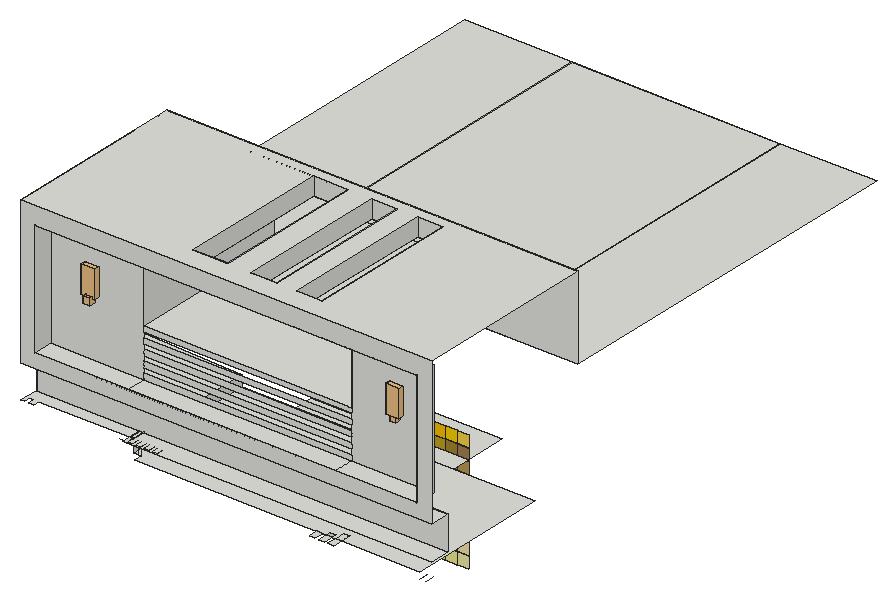
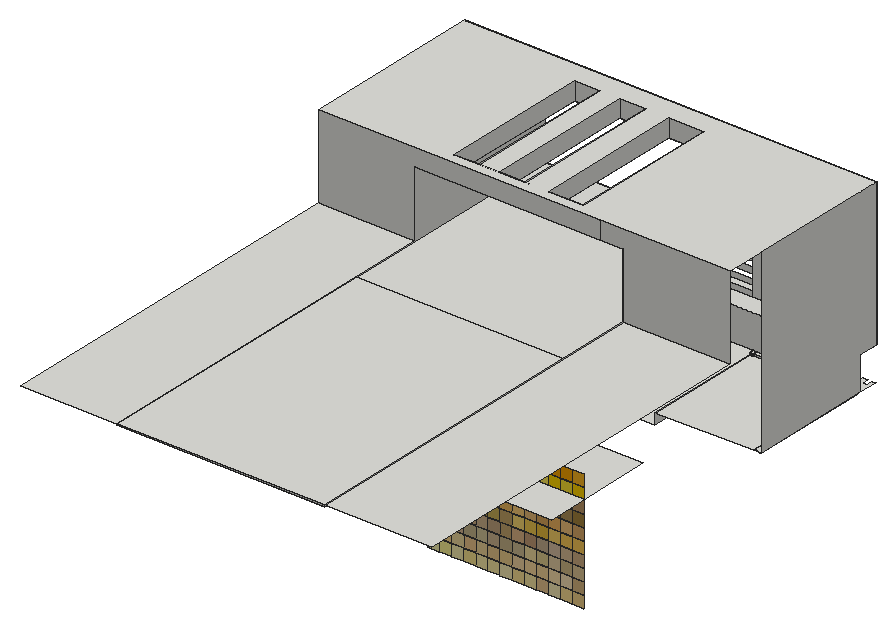
# SketchUp Ruby script. Lengths in inches.
U = 1.inch
M = Sketchup.active_model
def pt(a) = Geom::Point3d.new(a.map { |v| v * U })
def face(e, loops, mat)
  f = e.add_face(loops[0].map { |a| pt(a) })
  loops[1..].each { |l| e.add_face(l.map { |a| pt(a) }).erase! }
  f.material = f.back_material = mat if mat
  f
end
# faces: each face lists its corners as indices into pts; further lists are holes
def faces(e, pts, list, mat = nil) = list.each { |f| face(e, (f[0].is_a?(Array) ? f : [f]).map { |l| l.map { |i| pts[i] } }, mat) }
# xy, xz, yz: faces in a plane at the given z, y or x. An outline is a flat list of corners, or four numbers for a rectangle; further outlines are holes
def ring(l) = l.size == 4 ? [[l[0], l[1]], [l[2], l[1]], [l[2], l[3]], [l[0], l[3]]] : l.each_slice(2).to_a
def flat(e, list, mat, &to3) = list.each { |f| face(e, (f[0].is_a?(Array) ? f : [f]).map { |l| ring(l).map { |u, v| to3.(u, v) } }, mat) }
def xy(e, z, list, mat = nil) = flat(e, list, mat) { |x, y| [x, y, z] }
def xz(e, y, list, mat = nil) = flat(e, list, mat) { |x, z| [x, y, z] }
def yz(e, x, list, mat = nil) = flat(e, list, mat) { |y, z| [x, y, z] }
def lines(e, pts, list) = list.each { |a, b| e.add_line(pt(pts[a]), pt(pts[b])) }
# prism: a flat outline (further loops are holes) pulled along v
def prism(e, loops, v, mat = nil)
  f = face(e, loops, mat); d = Geom::Vector3d.new(v.map { |x| x * U })
  f.pushpull(f.normal.samedirection?(d) ? d.length : -d.length)
end
def box(e, o, s, mat = nil) = prism(e, [[o, [o[0] + s[0], o[1], o[2]], [o[0] + s[0], o[1] + s[1], o[2]], [o[0], o[1] + s[1], o[2]]]], [0, 0, s[2]], mat)
def at(x, y, z, deg = 0) = Geom::Transformation.translation(pt([x, y, z])) * Geom::Transformation.rotation(ORIGIN, Z_AXIS, deg.degrees)
def axes(o, x, y, z) = Geom::Transformation.new([*x, 0, *y, 0, *z, 0, *pt(o).to_a, 1])
def part(name) = M.definitions.add(name)
# library, detail: a bought-in or finely detailed component or shape, given as its bounding box
def library(name, o, s) = part(name).tap { |d| box(d.entities, o, s) }
def detail(e, o, s) = box(e.add_group.entities, o, s)
def put(e, d, t, mat = nil) = e.add_instance(d, t).tap { |i| i.material = mat if mat }
def group(e, t, mat = nil) = e.add_group.tap { |g| g.transformation = t; g.material = mat if mat }.entities
root = M.entities
M.materials.add("SW 0012 Empire Gold").color = [192, 162, 108]
M.materials.add("SW 0030 Colonial Yellow").color = [235, 202, 133]
M.materials.add("SW 0043 Peristyle Brass").color = [171, 151, 98]
M.materials.add("SW 0044 Hubbard Squash").color = [228, 196, 137]
M.materials.add("SW 0067 Belvedere Cream").color = [236, 208, 158]
M.materials.add("SW 0078 Sunbeam Yellow").color = [236, 216, 155]
M.materials.add("SW 2813 Downing Straw").color = [196, 173, 119]
M.materials.add("SW 2814 Rookwood Antique Gold").color = [158, 131, 78]
M.materials.add("SW 2817 Rookwood Amber").color = [185, 135, 62]
M.materials.add("SW 2831 Classical Gold").color = [230, 191, 112]
M.materials.add("SW 2834 Birdseye Maple").color = [221, 199, 142]
M.materials.add("SW 2853 New Colonial Yellow").color = [211, 178, 125]
M.materials.add("SW 2857 Peace Yellow").color = [231, 210, 153]
M.materials.add("SW 2858 Harvest Gold").color = [215, 167, 103]
M.materials.add("SW 2865 Classical Yellow").color = [244, 218, 144]
M.materials.add("SW 6114 Bagel").color = [213, 185, 146]
M.materials.add("SW 6115 Totally Tan").color = [202, 170, 129]
M.materials.add("SW 6116 Tatami Tan").color = [184, 148, 100]
M.materials.add("SW 6117 Smokey Topaz").color = [164, 127, 83]
M.materials.add("SW 6118 Leather Bound").color = [139, 102, 57]
M.materials.add("SW 6121 Whole Wheat").color = [203, 185, 145]
M.materials.add("SW 6122 Camelback").color = [194, 175, 133]
M.materials.add("SW 6123 Baguette").color = [175, 151, 103]
M.materials.add("SW 6128 Blonde").color = [217, 193, 145]
M.materials.add("SW 6129 Restrained Gold").color = [206, 183, 131]
M.materials.add("SW 6130 Mannered Gold").color = [189, 159, 99]
M.materials.add("SW 6131 Chamois").color = [172, 141, 84]
M.materials.add("SW 6132 Relic Bronze").color = [143, 113, 59]
M.materials.add("SW 6135 Ecru").color = [206, 193, 149]
M.materials.add("SW 6136 Harmonic Tan").color = [194, 179, 136]
M.materials.add("SW 6137 Burlap").color = [170, 155, 114]
M.materials.add("SW 6138 Artifact").color = [151, 136, 95]
M.materials.add("SW 6139 Mossy Gold").color = [124, 107, 64]
M.materials.add("SW 6366 Ambitious Amber").color = [238, 208, 148]
M.materials.add("SW 6367 Viva Gold").color = [227, 182, 114]
M.materials.add("SW 6368 Bakelite Gold").color = [212, 162, 89]
M.materials.add("SW 6369 Tassel").color = [195, 143, 67]
M.materials.add("SW 6370 Saucy Gold").color = [179, 122, 51]
M.materials.add("SW 6373 Harvester").color = [232, 201, 137]
M.materials.add("SW 6374 Torchlight").color = [226, 185, 106]
M.materials.add("SW 6375 Honeycomb").color = [210, 161, 84]
M.materials.add("SW 6376 Gold Coast").color = [195, 143, 57]
M.materials.add("SW 6377 Butterscotch").color = [180, 128, 52]
M.materials.add("SW 6380 Humble Gold").color = [232, 206, 147]
M.materials.add("SW 6381 Anjou Pear").color = [217, 181, 105]
M.materials.add("SW 6382 Ceremonial Gold").color = [208, 167, 85]
M.materials.add("SW 6383 Golden Rule").color = [199, 153, 65]
M.materials.add("SW 6384 Cut The Mustard").color = [182, 135, 47]
M.materials.add("SW 6388 Golden Fleece").color = [227, 182, 114]
M.materials.add("SW 6389 Butternut").color = [200, 164, 90]
M.materials.add("SW 6390 Bosc Pear").color = [188, 151, 83]
M.materials.add("SW 6391 Gallant Gold").color = [161, 128, 61]
M.materials.add("SW 6394 Sequin").color = [220, 200, 139]
M.materials.add("SW 6395 Alchemy").color = [197, 171, 86]
M.materials.add("SW 6396 Different Gold").color = [183, 156, 75]
M.materials.add("SW 6397 Nankeen").color = [162, 135, 46]
M.materials.add("SW 6398 Sconce Gold").color = [151, 121, 51]
M.materials.add("SW 6659 Captivating Cream").color = [243, 220, 176]
M.materials.add("SW 6660 Honey Blush").color = [243, 211, 152]
M.materials.add("SW 6661 Papaya").color = [238, 189, 120]
M.materials.add("SW 6662 Summer Day").color = [234, 176, 94]
M.materials.add("SW 6663 Saffron Thread").color = [223, 158, 74]
M.materials.add("SW 6666 Enjoyable Yellow").color = [244, 218, 167]
M.materials.add("SW 6667 Afterglow").color = [243, 209, 138]
M.materials.add("SW 6668 Sunrise").color = [242, 197, 116]
M.materials.add("SW 6669 Yarrow").color = [231, 180, 89]
M.materials.add("SW 6670 Gold Crest").color = [221, 159, 46]
M.materials.add("SW 6671 Curry").color = [214, 148, 38]
M.materials.add("SW 6673 Banana Cream").color = [243, 226, 174]
M.materials.add("SW 6674 Jonquil").color = [244, 216, 142]
M.materials.add("SW 6675 Afternoon").color = [248, 209, 116]
M.materials.add("SW 6676 Butterfield").color = [244, 196, 86]
M.materials.add("SW 6677 Goldenrod").color = [244, 196, 86]
M.materials.add("SW 6678 Sunflower").color = [223, 162, 35]
M.materials.add("SW 6680 Friendly Yellow").color = [241, 228, 176]
M.materials.add("SW 6681 Butter Up").color = [243, 225, 159]
M.materials.add("SW 6682 June Day").color = [242, 210, 111]
M.materials.add("SW 6683 Bee").color = [235, 196, 79]
M.materials.add("SW 6684 Brittlebush").color = [228, 184, 61]
M.materials.add("SW 6685 Trinket").color = [209, 161, 37]
M.materials.add("SW 6687 Lantern Light").color = [241, 228, 173]
M.materials.add("SW 6688 Solaria").color = [242, 221, 140]
M.materials.add("SW 6689 Overjoy").color = [233, 203, 89]
M.materials.add("SW 6690 Gambol Gold").color = [220, 186, 63]
M.materials.add("SW 6691 Glitzy Gold").color = [208, 168, 18]
M.materials.add("SW 6692 Auric").color = [191, 145, 0]
M.materials.add("SW 6694 Glad Yellow").color = [240, 230, 169]
M.materials.add("SW 6695 Midday").color = [242, 222, 135]
M.materials.add("SW 6696 Quilt Gold").color = [227, 203, 95]
M.materials.add("SW 6697 Nugget").color = [211, 184, 67]
M.materials.add("SW 6698 Kingdom Gold").color = [202, 173, 37]
M.materials.add("SW 6699 Crispy Gold").color = [191, 161, 37]
M.materials.add("SW 6888 Pizazz Peach").color = [243, 202, 146]
M.materials.add("SW 6889 Stirring Orange").color = [243, 181, 96]
M.materials.add("SW 6890 Osage Orange").color = [243, 166, 60]
M.materials.add("SW 6894 Forceful Orange").color = [242, 160, 0]
M.materials.add("SW 6895 Laughing Orange").color = [242, 160, 0]
M.materials.add("SW 6896 Solé").color = [243, 226, 157]
M.materials.add("SW 6897 Sundance").color = [245, 206, 103]
M.materials.add("SW 6898 Social Butterfly").color = [247, 193, 71]
M.materials.add("SW 6899 Nasturtiumb").color = [246, 178, 33]
M.materials.add("SW 6900 Optimistic Yellow").color = [242, 228, 163]
M.materials.add("SW 6901 Daffodil").color = [246, 223, 119]
M.materials.add("SW 6902 Decisive Yellow").color = [248, 211, 68]
M.materials.add("SW 6903 Cheerful").color = [250, 208, 0]
M.materials.add("SW 6904 Gusto Gold").color = [245, 181, 0]
M.materials.add("SW 6905 Goldfinch").color = [249, 192, 0]
M.materials.add("SW 6906 Citrus").color = [251, 205, 0]
M.materials.add("SW 6907 Forsythia").color = [251, 210, 0]
M.materials.add("SW 6908 Fun Yellow").color = [242, 235, 145]
M.materials.add("SW 6909 Lemon Twist").color = [248, 227, 86]
M.materials.add("SW 6910 Daisy").color = [246, 220, 49]
M.materials.add("SW 6911 Confident Yellow").color = [245, 214, 0]
M.materials.add("SW 6912 Glisten Yellow").color = [240, 235, 169]
M.materials.add("SW 7677 Gold Vessel").color = [233, 187, 138]
M.materials.add("SW 7679 Golden Gate").color = [217, 176, 132]
M.materials.add("SW 7680 Lanyard").color = [191, 153, 116]
M.materials.add("SW 7682 Bee_s Wax").color = [233, 192, 136]
M.materials.add("SW 7685 White Raisin").color = [228, 192, 140]
M.materials.add("SW 7689 Row House Tan").color = [211, 187, 159]
M.materials.add("SW 7690 Townhall Tan").color = [194, 171, 140]
M.materials.add("SW 7691 Biltmore Buff").color = [225, 202, 161]
M.materials.add("SW 7692 Cupola Yellow").color = [219, 188, 144]
M.materials.add("SW 7693 Stonebriar").color = [203, 172, 128]
M.materials.add("SW 7694 Dromedary Camel").color = [203, 175, 136]
M.materials.add("SW 7695 Mesa Tan").color = [190, 160, 124]
M.materials.add("SW 7697 Safari").color = [203, 179, 141]
M.materials.add("SW 7699 Rustic City").color = [188, 160, 113]
M.materials.add("SW 7700 Olde World Gold").color = [145, 116, 76]
M.materials.add("SW 7717 Ligonier Tan").color = [211, 178, 143]
c1 = library("Spot Light",[-5.1,-5.1,-11.05],[10.2,10.2,11.05])
c2 = library("WALL+LIGHT+74",[0,0,0],[5,2.75,10.11])
xy(root,1472.71,[[1349.53,376.08,1604.22,561.95]])
xy(root,1534.95,[[1638.86,127.85,1648.04,143.16],[1654.29,127.85,1663.98,143.16],[1669.29,127.85,1678.97,143.16],[1343.63,143.16,1343.63,155.91,1330.44,155.91,1330.44,376.08,1805.83,376.08,1805.83,143.16,1678.97,143.16,1678.97,158.47,1669.29,158.47,1669.29,143.16],[1669.29,143.16,1678.97,158.47]])
xy(root,1552.52,[[1324.51,155.91,1330.44,183.72]])
xy(root,1555.875,[[1324.16,143.16,1330.44,143.16,1330.44,144.72,1329.57,144.72,1329.57,155.91,1324.61,155.91,1324.61,144.72,1324.16,144.72],[1330.44,143.16,1824.45,176.1],[1157.08,144.72,1162.44,144.72,1162.44,155.91,1169.07,155.91,1169.07,144.72,1177.49,144.72,1177.49,155.91,1324.16,155.91,1324.16,176.1,1157.08,176.1],[1324.16,144.72,1324.61,155.91],[1329.57,144.72,1330.44,155.91],
  [1324.16,155.91,1324.51,176.1],[1324.51,155.91,1330.44,176.1],[1157.08,176.1,1324.16,183.72],[1324.16,176.1,1324.51,183.72],[1324.51,176.1,1330.44,183.72],
  [1157.08,183.72,1169.07,376.08]])
xy(root,1610.73,[[1157.08,143.16,1824.45,176.1]])
xy(root,1632.93,[[1180.77,143.16,1330.44,176.1],[1330.44,143.16,1668.23,176.1],[1668.23,143.16,1801.375,176.1]])
xy(root,1710.73,[[1330.44,176.1,1668.23,1046.1]])
xy(root,1712.64,[[1157.08,440.47,1330.44,1046.1],[1668.23,440.47,1824.45,1046.1],[1330.44,559.91,1668.23,1046.1]])
xy(root,1819.39,[[1180.77,143.16,1330.44,176.1],[[1330.44,143.16,1668.23,440.47],[1409.23,179.04,1464.89,422.71],[1503.31,179.04,1544.96,422.71],[1578.01,179.04,1618.61,422.71]],[1668.23,143.16,1801.375,176.1]])
xy(root,1847.8125,[[1157.08,143.16,1824.45,143.16,1824.45,440.47,1157.08,440.47,1157.08,422.71,1618.61,422.71,1618.61,179.04,1578.01,179.04,1578.01,422.71,1544.96,422.71,1544.96,179.04,1503.31,179.04,1503.31,422.71,1464.89,422.71,1464.89,179.04,1409.23,179.04,1409.23,422.71,1157.08,422.71]])
xz(root,143.16,[[1654.29,1534.95,1663.98,1534.95,1669.6,1540.4375,1659.92,1540.4375],[[1157.08,1610.73,1824.45,1847.8125],[1180.77,1632.93,1801.375,1819.39]]])
xz(root,155.91,[[1324.51,1552.52,1324.61,1555.875],[1324.61,1552.52,1329.57,1555.875],[1329.57,1552.52,1330.44,1555.875]])
xz(root,176.1,[[1157.08,1555.875,1824.45,1610.73],[1180.77,1632.93,1330.44,1819.39],[1330.44,1632.93,1668.23,1641.91],[1668.23,1632.93,1801.375,1819.39],[1330.44,1650.41,1668.23,1659.61],
  [1330.44,1667.76,1668.23,1677.2],[1330.44,1685.36,1668.23,1694.08],[1330.44,1702.53,1668.23,1710.73]])
xz(root,179.04,[[1409.23,1819.39,1464.89,1847.8125],[1503.31,1819.39,1544.96,1847.8125],[1578.01,1819.39,1618.61,1847.8125]])
xz(root,183.72,[[1324.51,1552.52,1324.51,1552.63,1330.44,1552.52],[1330.44,1552.52,1324.51,1552.63,1324.51,1555.875,1330.44,1555.875],[1324.51,1552.63,1324.16,1552.64,1324.16,1555.875,1324.51,1555.875],[1324.16,1552.64,1169.07,1555.64,1169.07,1555.875,1324.16,1555.875]])
xz(root,376.08,[[1169.07,1555.64,1169.07,1555.875,1157.08,1555.875]])
xz(root,422.71,[[1409.23,1819.39,1464.89,1847.8125],[1503.31,1819.39,1544.96,1847.8125],[1578.01,1819.39,1618.61,1847.8125]])
xz(root,440.47,[[1157.08,1712.64,1157.08,1847.8125,1368.23,1847.8125,1368.23,1819.39,1330.44,1819.39,1330.44,1712.64],[1668.23,1712.64,1668.23,1819.39,1368.23,1819.39,1368.23,1847.8125,1824.45,1847.8125,1824.45,1712.64]])
xz(root,494.58,[[1467.96,1372.2,1486.61,1390.85]],"SW 0012 Empire Gold")
xz(root,494.58,[[1350.34,1313.39,1369,1332.04]],"SW 0030 Colonial Yellow")
xz(root,494.58,[[1467.96,1431,1486.61,1449.66]],"SW 0043 Peristyle Brass")
xz(root,494.58,[[1487.56,1332.99,1506.21,1351.65]],"SW 0044 Hubbard Squash")
xz(root,494.58,[[1448.35,1332.99,1467.01,1351.65]],"SW 0067 Belvedere Cream")
xz(root,494.58,[[1428.75,1352.6,1447.4,1371.25]],"SW 0078 Sunbeam Yellow")
xz(root,494.58,[[1507.16,1431,1525.8125,1449.66]],"SW 2813 Downing Straw")
xz(root,494.58,[[1389.55,1431,1408.2,1449.66]],"SW 2814 Rookwood Antique Gold")
xz(root,494.58,[[1389.55,1450.61,1408.2,1469.26]],"SW 2817 Rookwood Amber")
xz(root,494.58,[[1507.16,1411.4,1525.8125,1430.05]],"SW 2831 Classical Gold")
xz(root,494.58,[[1565.97,1372.2,1584.62,1390.85]],"SW 2834 Birdseye Maple")
xz(root,494.58,[[1350.34,1332.99,1369,1351.65]],"SW 2853 New Colonial Yellow")
xz(root,494.58,[[1546.36,1332.99,1565.02,1351.65]],"SW 2857 Peace Yellow")
xz(root,494.58,[[1350.34,1411.4,1369,1430.05]],"SW 2858 Harvest Gold")
xz(root,494.58,[[1448.35,1313.39,1467.01,1332.04]],"SW 2865 Classical Yellow")
xz(root,494.58,[[1369.95,1372.2,1388.6,1390.85]],"SW 6114 Bagel")
xz(root,494.58,[[1350.34,1372.2,1369,1390.85]],"SW 6115 Totally Tan")
xz(root,494.58,[[1350.34,1450.61,1369,1469.26]],"SW 6116 Tatami Tan")
xz(root,494.58,[[1585.57,1470.21,1604.22,1488.86]],"SW 6117 Smokey Topaz")
xz(root,494.58,[[1369.95,1450.61,1388.6,1469.26]],"SW 6118 Leather Bound")
xz(root,494.58,[[1448.35,1352.6,1467.01,1371.25]],"SW 6121 Whole Wheat")
xz(root,494.58,[[1467.96,1352.6,1486.61,1371.25]],"SW 6122 Camelback")
xz(root,494.58,[[1428.75,1431,1447.4,1449.66]],"SW 6123 Baguette")
xz(root,494.58,[[1350.34,1352.6,1369,1371.25]],"SW 6128 Blonde")
xz(root,494.58,[[1369.95,1352.6,1388.6,1371.25]],"SW 6129 Restrained Gold")
xz(root,494.58,[[1467.96,1391.8,1486.61,1410.45]],"SW 6130 Mannered Gold")
xz(root,494.58,[[1369.95,1431,1388.6,1449.66]],"SW 6131 Chamois")
xz(root,494.58,[[1409.15,1431,1427.8,1449.66]],"SW 6132 Relic Bronze")
xz(root,494.58,[[1507.16,1352.6,1525.8125,1371.25]],"SW 6135 Ecru")
xz(root,494.58,[[1526.76,1352.6,1545.41,1371.25]],"SW 6136 Harmonic Tan")
xz(root,494.58,[[1546.36,1431,1565.02,1449.66]],"SW 6137 Burlap")
xz(root,494.58,[[1565.97,1431,1584.62,1449.66]],"SW 6138 Artifact")
xz(root,494.58,[[1585.57,1431,1604.22,1449.66]],"SW 6139 Mossy Gold")
xz(root,494.58,[[1409.15,1332.99,1427.8,1351.65]],"SW 6366 Ambitious Amber")
xz(root,494.58,[[1428.75,1411.4,1447.4,1430.05]],"SW 6367 Viva Gold")
xz(root,494.58,[[1409.15,1411.4,1427.8,1430.05]],"SW 6368 Bakelite Gold")
xz(root,494.58,[[1409.15,1450.61,1427.8,1469.26]],"SW 6369 Tassel")
xz(root,494.58,[[1428.75,1450.61,1447.4,1469.26]],"SW 6370 Saucy Gold")
xz(root,494.58,[[1467.96,1332.99,1486.61,1351.65]],"SW 6373 Harvester")
xz(root,494.58,[[1487.56,1411.4,1506.21,1430.05]],"SW 6374 Torchlight")
xz(root,494.58,[[1526.76,1411.4,1545.41,1430.05]],"SW 6375 Honeycomb")
xz(root,494.58,[[1467.96,1450.61,1486.61,1469.26]],"SW 6376 Gold Coast")
xz(root,494.58,[[1448.35,1450.61,1467.01,1469.26]],"SW 6377 Butterscotch")
xz(root,494.58,[[1507.16,1332.99,1525.8125,1351.65]],"SW 6380 Humble Gold")
xz(root,494.58,[[1546.36,1411.4,1565.02,1430.05]],"SW 6381 Anjou Pear")
xz(root,494.58,[[1487.56,1450.61,1506.21,1469.26]],"SW 6382 Ceremonial Gold")
xz(root,494.58,[[1507.16,1450.61,1525.8125,1469.26]],"SW 6383 Golden Rule")
xz(root,494.58,[[1526.76,1450.61,1545.41,1469.26]],"SW 6384 Cut The Mustard")
xz(root,494.58,[[1585.57,1372.2,1604.22,1390.85]],"SW 6388 Golden Fleece")
xz(root,494.58,[[1565.97,1450.61,1584.62,1469.26]],"SW 6389 Butternut")
xz(root,494.58,[[1585.57,1450.61,1604.22,1469.26]],"SW 6390 Bosc Pear")
xz(root,494.58,[[1350.34,1431,1369,1449.66]],"SW 6391 Gallant Gold")
xz(root,494.58,[[1409.15,1352.6,1427.8,1371.25]],"SW 6394 Sequin")
xz(root,494.58,[[1487.56,1391.8,1506.21,1410.45]],"SW 6395 Alchemy")
xz(root,494.58,[[1507.16,1391.8,1525.8125,1410.45]],"SW 6396 Different Gold")
xz(root,494.58,[[1565.97,1470.21,1584.62,1488.86]],"SW 6397 Nankeen")
xz(root,494.58,[[1526.76,1431,1545.41,1449.66]],"SW 6398 Sconce Gold")
xz(root,494.58,[[1369.95,1332.99,1388.6,1351.65]],"SW 6659 Captivating Cream")
xz(root,494.58,[[1428.75,1332.99,1447.4,1351.65]],"SW 6660 Honey Blush")
xz(root,494.58,[[1369.95,1411.4,1388.6,1430.05]],"SW 6661 Papaya")
xz(root,494.58,[[1389.55,1411.4,1408.2,1430.05]],"SW 6662 Summer Day")
xz(root,494.58,[[1448.35,1489.81,1467.01,1508.46]],"SW 6663 Saffron Thread")
xz(root,494.58,[[1389.55,1332.99,1408.2,1351.65]],"SW 6666 Enjoyable Yellow")
xz(root,494.58,[[1565.97,1332.99,1584.62,1351.65]],"SW 6667 Afterglow")
xz(root,494.58,[[1448.35,1411.4,1467.01,1430.05]],"SW 6668 Sunrise")
xz(root,494.58,[[1467.96,1411.4,1486.61,1430.05]],"SW 6669 Yarrow")
xz(root,494.58,[[1487.56,1489.81,1506.21,1508.46]],"SW 6670 Gold Crest")
xz(root,494.58,[[1467.96,1489.81,1486.61,1508.46]],"SW 6671 Curry")
xz(root,494.58,[[1585.57,1332.99,1604.22,1351.65]],"SW 6673 Banana Cream")
xz(root,494.58,[[1369.95,1313.39,1388.6,1332.04]],"SW 6674 Jonquil")
xz(root,494.58,[[1565.97,1411.4,1584.62,1430.05]],"SW 6675 Afternoon")
xz(root,494.58,[[1350.34,1391.8,1369,1410.45]],"SW 6676 Butterfield")
xz(root,494.58,[[1369.95,1391.8,1388.6,1410.45]],"SW 6677 Goldenrod")
xz(root,494.58,[[1507.16,1489.81,1525.8125,1508.46]],"SW 6678 Sunflower")
xz(root,494.58,[[1389.55,1313.39,1408.2,1332.04]],"SW 6680 Friendly Yellow")
xz(root,494.58,[[1428.75,1313.39,1447.4,1332.04]],"SW 6681 Butter Up")
xz(root,494.58,[[1448.35,1391.8,1467.01,1410.45]],"SW 6682 June Day")
xz(root,494.58,[[1428.75,1391.8,1447.4,1410.45]],"SW 6683 Bee")
xz(root,494.58,[[1409.15,1391.8,1427.8,1410.45]],"SW 6684 Brittlebush")
xz(root,494.58,[[1546.36,1450.61,1565.02,1469.26]],"SW 6685 Trinket")
xz(root,494.58,[[1467.96,1313.39,1486.61,1332.04]],"SW 6687 Lantern Light")
xz(root,494.58,[[1526.76,1313.39,1545.41,1332.04]],"SW 6688 Solaria")
xz(root,494.58,[[1546.36,1391.8,1565.02,1410.45]],"SW 6689 Overjoy")
xz(root,494.58,[[1448.35,1470.21,1467.01,1488.86]],"SW 6690 Gambol Gold")
xz(root,494.58,[[1467.96,1470.21,1486.61,1488.86]],"SW 6691 Glitzy Gold")
xz(root,494.58,[[1487.56,1470.21,1506.21,1488.86]],"SW 6692 Auric")
xz(root,494.58,[[1546.36,1313.39,1565.02,1332.04]],"SW 6694 Glad Yellow")
xz(root,494.58,[[1526.76,1391.8,1545.41,1410.45]],"SW 6695 Midday")
xz(root,494.58,[[1565.97,1391.8,1584.62,1410.45]],"SW 6696 Quilt Gold")
xz(root,494.58,[[1507.16,1470.21,1525.8125,1488.86]],"SW 6697 Nugget")
xz(root,494.58,[[1526.76,1470.21,1545.41,1488.86]],"SW 6698 Kingdom Gold")
xz(root,494.58,[[1546.36,1470.21,1565.02,1488.86]],"SW 6699 Crispy Gold")
xz(root,494.58,[[1565.97,1352.6,1584.62,1371.25]],"SW 6888 Pizazz Peach")
xz(root,494.58,[[1428.75,1489.81,1447.4,1508.46]],"SW 6889 Stirring Orange")
xz(root,494.58,[[1409.15,1489.81,1427.8,1508.46]],"SW 6890 Osage Orange")
xz(root,494.58,[[1389.55,1489.81,1408.2,1508.46]],"SW 6894 Forceful Orange")
xz(root,494.58,[[1369.95,1489.81,1388.6,1508.46]],"SW 6895 Laughing Orange")
xz(root,494.58,[[1487.56,1313.39,1506.21,1332.04]],"SW 6896 Solé")
xz(root,494.58,[[1389.55,1391.8,1408.2,1410.45]],"SW 6897 Sundance")
xz(root,494.58,[[1585.57,1411.4,1604.22,1430.05]],"SW 6898 Social Butterfly")
xz(root,494.58,[[1350.34,1489.81,1369,1508.46]],"SW 6899 Nasturtiumb")
xz(root,494.58,[[1507.16,1313.39,1525.8125,1332.04]],"SW 6900 Optimistic Yellow")
xz(root,494.58,[[1585.57,1391.8,1604.22,1410.45]],"SW 6901 Daffodil")
xz(root,494.58,[[1585.57,1489.81,1604.22,1508.46]],"SW 6902 Decisive Yellow")
xz(root,494.58,[[1565.97,1489.81,1584.62,1508.46]],"SW 6903 Cheerful")
xz(root,494.58,[[1526.76,1489.81,1545.41,1508.46]],"SW 6904 Gusto Gold")
xz(root,494.58,[[1546.36,1489.81,1565.02,1508.46]],"SW 6905 Goldfinch")
xz(root,494.58,[[1350.34,1470.21,1369,1488.86]],"SW 6906 Citrus")
xz(root,494.58,[[1389.55,1470.21,1408.2,1488.86]],"SW 6907 Forsythia")
xz(root,494.58,[[1565.97,1313.39,1584.62,1332.04]],"SW 6908 Fun Yellow")
xz(root,494.58,[[1409.15,1470.21,1427.8,1488.86]],"SW 6909 Lemon Twist")
xz(root,494.58,[[1369.95,1470.21,1388.6,1488.86]],"SW 6910 Daisy")
xz(root,494.58,[[1428.75,1470.21,1447.4,1488.86]],"SW 6911 Confident Yellow")
xz(root,494.58,[[1585.57,1313.39,1604.22,1332.04]],"SW 6912 Glisten Yellow")
xz(root,494.58,[[1585.57,1352.6,1604.22,1371.25]],"SW 7677 Gold Vessel")
xz(root,494.58,[[1448.35,1372.2,1467.01,1390.85]],"SW 7679 Golden Gate")
xz(root,494.58,[[1428.75,1372.2,1447.4,1390.85]],"SW 7680 Lanyard")
xz(root,494.58,[[1526.76,1332.99,1545.41,1351.65]],"SW 7682 Bee_s Wax")
xz(root,494.58,[[1409.15,1313.39,1427.8,1332.04]],"SW 7685 White Raisin")
xz(root,494.58,[[1389.55,1372.2,1408.2,1390.85]],"SW 7689 Row House Tan")
xz(root,494.58,[[1409.15,1372.2,1427.8,1390.85]],"SW 7690 Townhall Tan")
xz(root,494.58,[[1389.55,1352.6,1408.2,1371.25]],"SW 7691 Biltmore Buff")
xz(root,494.58,[[1546.36,1372.2,1565.02,1390.85]],"SW 7692 Cupola Yellow")
xz(root,494.58,[[1526.76,1372.2,1545.41,1390.85]],"SW 7693 Stonebriar")
xz(root,494.58,[[1507.16,1372.2,1525.8125,1390.85]],"SW 7694 Dromedary Camel")
xz(root,494.58,[[1487.56,1372.2,1506.21,1390.85]],"SW 7695 Mesa Tan")
xz(root,494.58,[[1487.56,1352.6,1506.21,1371.25]],"SW 7697 Safari")
xz(root,494.58,[[1487.56,1431,1506.21,1449.66]],"SW 7699 Rustic City")
xz(root,494.58,[[1448.35,1431,1467.01,1449.66]],"SW 7700 Olde World Gold")
xz(root,494.58,[[1546.36,1352.6,1565.02,1371.25]],"SW 7717 Ligonier Tan")
xz(root,1046.1,[[1330.44,1710.73,1668.23,1712.64]])
yz(root,1157.08,[[176.1,1555.875,176.1,1610.73,143.16,1610.73,143.16,1847.8125,376.08,1847.8125,376.08,1555.875]])
yz(root,1169.07,[[183.72,1555.64,376.08,1555.875]])
yz(root,1180.77,[[143.16,1632.93,176.1,1819.39]])
yz(root,1324.51,[[155.91,1552.52,183.72,1555.875]])
yz(root,1330.44,[[155.91,1534.95,183.72,1552.52],[183.72,1534.95,376.08,1552.52],[155.91,1552.52,183.72,1555.875],[176.1,1710.73,1046.1,1710.73,1046.1,1712.64,440.47,1712.64,440.47,1819.39,176.1,1819.39]])
yz(root,1409.23,[[179.04,1819.39,422.71,1847.8125]])
yz(root,1464.89,[[179.04,1819.39,422.71,1847.8125]])
yz(root,1503.31,[[179.04,1819.39,422.71,1847.8125]])
yz(root,1544.96,[[179.04,1819.39,422.71,1847.8125]])
yz(root,1578.01,[[179.04,1819.39,422.71,1847.8125]])
yz(root,1618.61,[[179.04,1819.39,422.71,1847.8125]])
yz(root,1668.23,[[176.1,1710.73,176.1,1819.39,440.47,1819.39,440.47,1712.64,1046.1,1712.64,1046.1,1710.73]])
yz(root,1801.375,[[143.16,1632.93,176.1,1819.39]])
p = [[1169.07,376.08,1555.64],[1330.44,376.08,1552.52],[1330.44,183.72,1552.52],[1324.51,183.72,1552.63],[1324.16,183.72,1552.64],[1169.07,183.72,1555.64],
  [1316.19,144.72,1555.875],[1324.16,144.72,1555.875],[1337.99,155.91,1555.875],[1337.99,155.91,1534.95],[1337.99,144.72,1555.875],[1330.44,144.72,1555.875],
  [1351.36,155.91,1555.875],[1351.36,144.72,1555.875],[1342.94,155.91,1555.875],[1342.94,144.72,1555.875],[1342.94,155.91,1534.95],[1364.74,155.91,1555.875],
  [1364.74,144.72,1555.875],[1356.32,155.91,1555.875],[1356.32,144.72,1555.875],[1378.11,155.91,1555.875],[1378.11,144.72,1555.875],[1369.69,155.91,1555.875],
  [1369.69,144.72,1555.875],[1817.79,143.16,1534.95],[1817.79,127.85,1534.95],[1827.47,143.16,1534.95],[1827.47,127.85,1534.95]]
faces(root,p,[[0,1,2,3,4,5]])
lines(root,p,[[6,7],[8,9],[8,10],[11,10],[12,13],[14,15],[15,13],[16,14],[17,18],[19,20],[20,18],[21,22],
  [23,24],[24,22],[25,26],[27,28]])
put(root,c1,at(1248.61,168,1730.28))
put(root,c1,at(1741.98,173.44,1730.28))
put(root,c2,axes([1236.79,167.23,1727.84],[4.342,0,0],[0,4.342,0],[0,0,4.342]))
put(root,c2,axes([1730.67,167.23,1727.84],[4.342,0,0],[0,4.342,0],[0,0,4.342]))
